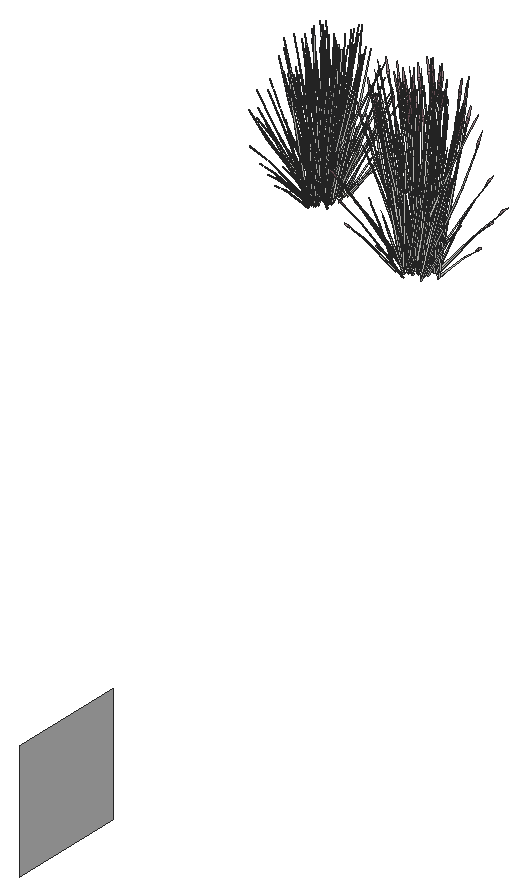
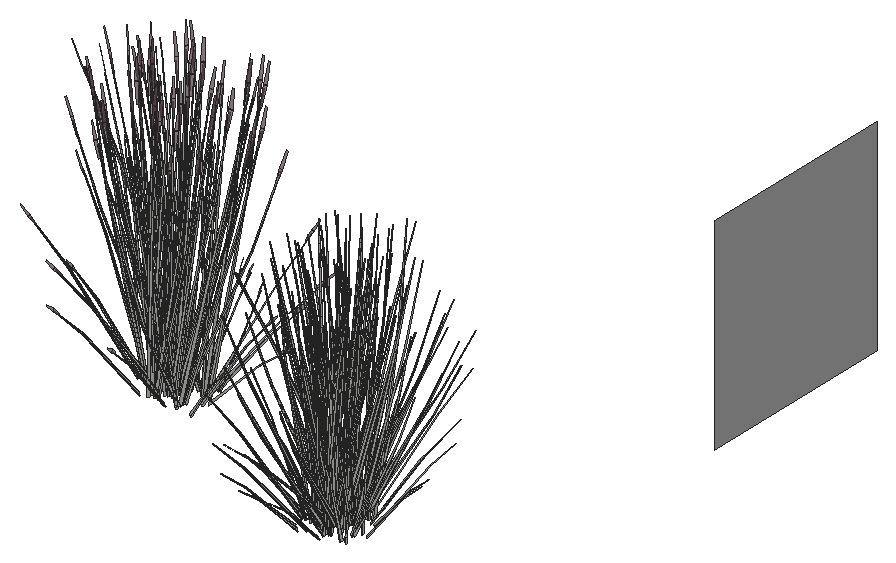
# SketchUp Ruby script. Lengths in inches.
U = 1.inch
M = Sketchup.active_model
def pt(a) = Geom::Point3d.new(a.map { |v| v * U })
def face(e, loops, mat)
  f = e.add_face(loops[0].map { |a| pt(a) })
  loops[1..].each { |l| e.add_face(l.map { |a| pt(a) }).erase! }
  f.material = f.back_material = mat if mat
  f
end
# faces: each face lists its corners as indices into pts; further lists are holes
def faces(e, pts, list, mat = nil) = list.each { |f| face(e, (f[0].is_a?(Array) ? f : [f]).map { |l| l.map { |i| pts[i] } }, mat) }
# xy, xz, yz: faces in a plane at the given z, y or x. An outline is a flat list of corners, or four numbers for a rectangle; further outlines are holes
def ring(l) = l.size == 4 ? [[l[0], l[1]], [l[2], l[1]], [l[2], l[3]], [l[0], l[3]]] : l.each_slice(2).to_a
def flat(e, list, mat, &to3) = list.each { |f| face(e, (f[0].is_a?(Array) ? f : [f]).map { |l| ring(l).map { |u, v| to3.(u, v) } }, mat) }
def xy(e, z, list, mat = nil) = flat(e, list, mat) { |x, y| [x, y, z] }
def xz(e, y, list, mat = nil) = flat(e, list, mat) { |x, z| [x, y, z] }
def yz(e, x, list, mat = nil) = flat(e, list, mat) { |y, z| [x, y, z] }
def lines(e, pts, list) = list.each { |a, b| e.add_line(pt(pts[a]), pt(pts[b])) }
# prism: a flat outline (further loops are holes) pulled along v
def prism(e, loops, v, mat = nil)
  f = face(e, loops, mat); d = Geom::Vector3d.new(v.map { |x| x * U })
  f.pushpull(f.normal.samedirection?(d) ? d.length : -d.length)
end
def box(e, o, s, mat = nil) = prism(e, [[o, [o[0] + s[0], o[1], o[2]], [o[0] + s[0], o[1] + s[1], o[2]], [o[0], o[1] + s[1], o[2]]]], [0, 0, s[2]], mat)
def at(x, y, z, deg = 0) = Geom::Transformation.translation(pt([x, y, z])) * Geom::Transformation.rotation(ORIGIN, Z_AXIS, deg.degrees)
def axes(o, x, y, z) = Geom::Transformation.new([*x, 0, *y, 0, *z, 0, *pt(o).to_a, 1])
def part(name) = M.definitions.add(name)
# library, detail: a bought-in or finely detailed component or shape, given as its bounding box
def library(name, o, s) = part(name).tap { |d| box(d.entities, o, s) }
def detail(e, o, s) = box(e.add_group.entities, o, s)
def put(e, d, t, mat = nil) = e.add_instance(d, t).tap { |i| i.material = mat if mat }
def group(e, t, mat = nil) = e.add_group.tap { |g| g.transformation = t; g.material = mat if mat }.entities
root = M.entities
M.materials.add("Glass_Mirror_01").color = [185, 185, 185]
M.materials.add("LightPink_Translucent").color = [144, 107, 117]
M.materials["LightPink_Translucent"].alpha = 0.75
c1 = part("blade")
p = [[2.15,0.21,22],[0,0.17,0],[0.09,0.45,0],[2.18,0.31,22],[2.29,0.31,22],[0.38,0.45,0],
  [2.48,0.24,33],[2.49,0.24,33],[2.48,0.22,33]]
faces(c1.entities,p,[[0,1,2,3],[4,5,2,3],[6,3,4,7],[8,0,3,6]])
c2 = part("blade with seeds\#1")
put(c2.entities,c1,at(0,0,0))
c3 = part("seeds")
p = [[0.3,-0.1,1.38],[-0.01,-0.03,1.59],[-0.01,-0.03,0.03],[0.14,-0.07,-0.07],[0.29,-0.03,3],[0.15,0.01,3.11]]
faces(c3.entities,p,[[0,1,2,3],[1,0,4,5]],"LightPink_Translucent")
c4 = part("blade with seeds")
put(c4.entities,c1,at(0,0,0))
put(c4.entities,c3,axes([2.4,0.25,30.99],[1.5799,-0.05474,1.17369],[-0.12525,1.92788,0.29478],[-0.07173,-0.02425,1.56792]))
yz(root,291,[[55.83,53.72,96.48,94.93]],"Glass_Mirror_01")
put(root,c2,axes([219.63,280.1875,145.32],[-1.0019,0.47479,-0.62955],[-0.36083,-1.36768,-0.16523],[-0.33927,0.05248,1.38963]))
put(root,c2,axes([221.34,275.85,145.32],[0.89455,-0.42392,-0.62393],[0.32217,1.22114,-0.16376],[0.30292,-0.04686,1.37722]))
put(root,c2,axes([219.46,275.97,145.28],[0.16018,-1.20264,-0.5621],[0.98808,0.25378,-0.14753],[0.11973,-0.3589,1.24074]))
put(root,c2,axes([221.5,280,145.28],[-0.16018,1.20264,-0.5621],[-0.98808,-0.25378,-0.14753],[-0.11973,0.3589,1.24074]))
put(root,c2,axes([218.61,278.11,145.28],[-0.73437,-0.77871,-0.5621],[0.66591,-0.96736,-0.14753],[-0.18319,-0.31204,1.24074]))
put(root,c2,axes([222.36,277.86,145.28],[0.73437,0.77871,-0.5621],[-0.66591,0.96736,-0.14753],[0.18319,0.31204,1.24074]))
put(root,c4,axes([263.91,261.5,146.02],[-0.50328,-1.06202,-0.69835],[1.44974,-0.38248,-0.18329],[-0.05563,-0.35963,1.54149]))
put(root,c4,axes([268.51,263.3,146.02],[0.44936,0.94823,-0.69212],[-1.29441,0.3415,-0.18165],[0.04967,0.32109,1.52773]))
put(root,c4,axes([268.38,261.3125,145.98],[1.27479,0.1698,-0.62353],[-0.26901,1.04736,-0.16365],[0.38043,0.12691,1.37633]))
put(root,c4,axes([264.11,263.48,145.98],[-1.27479,-0.1698,-0.62353],[0.26901,-1.04736,-0.16365],[-0.38043,-0.12691,1.37633]))
put(root,c4,axes([266.11,260.41,145.98],[0.82544,-0.77843,-0.62353],[1.0254,0.70586,-0.16365],[0.33076,-0.19418,1.37633]))
put(root,c4,axes([266.375,264.38,145.98],[-0.82544,0.77843,-0.62353],[-1.0254,-0.70586,-0.16365],[-0.33076,0.19418,1.37633]))
put(root,c2,axes([217.59,274.39,145.25],[0.48852,-1.08202,-0.44759],[0.87598,0.64674,0],[0.11126,-0.24644,1.41987]))
put(root,c2,axes([224.36,276.58,145.25],[0.48852,1.08202,-0.44759],[-0.87598,0.64674,0],[0.11126,0.24644,1.41987]))
put(root,c2,axes([219.49,282.99,145.25],[-0.97703,0,-0.44759],[0,-1.29348,0],[-0.22253,0,1.41987]))
put(root,c2,axes([223.375,281.58,145.25],[-0.48852,1.08202,-0.44759],[-0.87598,-0.64674,0],[-0.11126,0.24644,1.41987]))
put(root,c2,axes([216.6,279.39,145.25],[-0.48852,-1.08202,-0.44759],[0.87598,-0.64674,0],[-0.11126,-0.24644,1.41987]))
put(root,c2,axes([221.47,272.99,145.25],[0.97703,0,-0.44759],[0,1.29348,0],[0.22253,0,1.41987]))
put(root,c2,axes([219.89,279.47,145.42],[-0.88038,-0.56093,-0.40331],[0.4237,-1.16553,0.1941],[-0.20294,0,1.29492]))
put(root,c2,axes([221.1875,279.38,145.42],[-0.82007,0.69452,-0.40331],[-0.57748,-1.05199,0.1941],[-0.10147,0.22475,1.29492]))
put(root,c2,axes([219.77,276.59,145.42],[0.82007,-0.69452,-0.40331],[0.57748,1.05199,0.1941],[0.10147,-0.22475,1.29492]))
put(root,c2,axes([221.07,276.51,145.42],[0.88038,0.56093,-0.40331],[-0.4237,1.16553,0.1941],[0.20294,0,1.29492]))
put(root,c2,axes([221.78,277.9,145.42],[0.06031,1.25545,-0.40331],[-1.00118,0.11354,0.1941],[0.10147,0.22475,1.29492]))
put(root,c4,axes([270.05,259.33,145.94],[1.14694,0.51783,-0.49651],[-0.68554,0.92854,0],[0.26122,0.11794,1.57504]))
put(root,c4,axes([267.73,266.51,145.94],[-1.14694,0.51783,-0.49651],[-0.68554,-0.92854,0],[-0.26122,0.11794,1.57504]))
put(root,c4,axes([260.94,261.35,145.94],[0,-1.03566,-0.49651],[1.37109,0,0],[0,-0.23588,1.57504]))
put(root,c4,axes([262.43,265.46,145.94],[-1.14694,-0.51783,-0.49651],[0.68554,-0.92854,0],[-0.26122,-0.11794,1.57504]))
put(root,c4,axes([264.75,258.28,145.94],[1.14694,-0.51783,-0.49651],[0.68554,0.92854,0],[0.26122,-0.11794,1.57504]))
put(root,c4,axes([271.54,263.44,145.94],[0,1.03566,-0.49651],[-1.37109,0,0],[0,0.23588,1.57504]))
put(root,c2,axes([216.99,279.14,145.26],[0.24175,-1.0786,-0.27926],[0.85134,0.27158,0.27926],[-0.09817,-0.21744,1.25283]))
put(root,c2,axes([221.45,273.54,145.26],[0.60959,0.80703,-0.27926],[-0.60959,0.80703,0.27926],[0.19635,0,1.25283]))
put(root,c2,axes([223.01,281.28,145.26],[-0.85134,0.27158,-0.27926],[-0.24175,-1.0786,0.27926],[-0.09817,0.21744,1.25283]))
put(root,c2,axes([223.98,276.83,145.26],[-0.24175,1.0786,-0.27926],[-0.85134,-0.27158,0.27926],[0.09817,0.21744,1.25283]))
put(root,c2,axes([217.95,274.69,145.26],[0.85134,-0.27158,-0.27926],[0.24175,1.0786,0.27926],[0.09817,-0.21744,1.25283]))
put(root,c2,axes([219.52,282.43,145.26],[-0.60959,-0.80703,-0.27926],[0.60959,-0.80703,0.27926],[-0.19635,0,1.25283]))
put(root,c2,axes([224.54,274.45,144.77],[-0.14106,-0.08423,1.5897],[-0.41543,-1.06044,-0.24285],[0.21501,-0.3215,0.27078]))
put(root,c2,axes([220.11,283.87,144.77],[0.15398,-0.02932,1.5897],[0.80412,0.59108,-0.24285],[-0.04053,0.41985,0.27078]))
put(root,c2,axes([214.89,278.59,144.77],[0.0352,0.19392,1.5897],[-0.39624,1.07238,-0.24285],[-0.33051,-0.01799,0.27078]))
put(root,c2,axes([224.51,279.4,144.77],[-0.05317,-0.18711,1.5897],[0.29263,-1.12549,-0.24285],[0.32981,-0.03291,0.27078]))
put(root,c2,axes([220.26,271.39,144.77],[-0.14833,0.06042,1.5897],[-0.86768,-0.41907,-0.24285],[-0.01248,-0.42273,0.27078]))
put(root,c2,axes([216.1,282.05,144.77],[0.12871,0.11199,1.5897],[0.2775,1.13173,-0.24285],[-0.25244,0.2734,0.27078]))
put(root,c2,axes([224.42,284.18,144.77],[0.09761,-0.15508,1.5897],[0.90442,-0.26295,-0.24285],[0.19286,0.3437,0.27078]))
put(root,c2,axes([216.57,273.84,144.77],[-0.07697,0.17304,1.5897],[-0.85991,0.44448,-0.24285],[-0.23336,-0.29985,0.27078]))
put(root,c4,axes([264.67,261.77,146.13],[0.59459,-0.93321,-0.44739],[1.23546,0.44912,0.21531],[0,-0.21512,1.43643]))
put(root,c4,axes([264.77,263.15,146.13],[-0.73619,-0.86927,-0.44739],[1.11511,-0.61213,0.21531],[-0.23824,-0.10756,1.43643]))
put(root,c4,axes([267.72,261.65,146.13],[0.73619,0.86927,-0.44739],[-1.11511,0.61213,0.21531],[0.23824,0.10756,1.43643]))
put(root,c4,axes([267.8125,263.02,146.13],[-0.59459,0.93321,-0.44739],[-1.23546,-0.44912,0.21531],[0,0.21512,1.43643]))
put(root,c4,axes([266.34,263.77,146.13],[-1.33077,0.06393,-0.44739],[-0.12035,-1.06125,0.21531],[-0.23824,0.10756,1.43643]))
put(root,c2,axes([218.74,280.28,144.86],[0.39117,1.13797,1.16227],[-1.12236,0.3622,0.45161],[0.01867,-0.69878,1.32195]))
put(root,c2,axes([222.61,276.62,145.4],[-0.33151,-1.21377,-0.17307],[0.95493,-0.4265,0.00007],[-0.03664,-0.13398,1.56765]))
put(root,c2,axes([221.51,277.02,145.83],[1.11485,-0.13472,-0.26229],[0.06741,1.40314,-0.45076],[0.1485,0.24708,1.43974]))
put(root,c2,axes([220.34,276.37,145.83],[0.46619,-1.302,-0.26229],[0.98396,0.62692,-0.45076],[0.24158,-0.04092,1.43974]))
put(root,c2,axes([220.625,279.61,145.83],[-0.46619,1.302,-0.26229],[-0.98396,-0.62692,-0.45076],[-0.24158,0.04092,1.43974]))
put(root,c2,axes([219.46,278.95,145.83],[-1.11485,0.13472,-0.26229],[-0.06741,-1.40314,-0.45076],[-0.1485,-0.24708,1.43974]))
put(root,c2,axes([219.3125,277.33,145.83],[-0.64866,-1.16728,-0.26229],[0.91655,-0.77622,-0.45076],[0.09308,-0.288,1.43974]))
put(root,c2,axes([221.65,278.64,145.83],[0.64866,1.16728,-0.26229],[-0.91655,0.77622,-0.45076],[-0.09308,0.288,1.43974]))
put(root,c4,axes([265.02,258.69,145.95],[1.14332,0.25625,-0.30978],[-0.28787,0.90242,0.30978],[0.23049,-0.10406,1.38974]))
put(root,c4,axes([270.95,263.42,145.95],[-0.85545,0.64616,-0.30978],[-0.85545,-0.64616,0.30978],[0,0.20813,1.38974]))
put(root,c4,axes([262.75,265.07,145.95],[-0.28787,-0.90242,-0.30978],[1.14332,-0.25625,0.30978],[-0.23049,-0.10406,1.38974]))
put(root,c4,axes([267.46,266.1,145.95],[-1.14332,-0.25625,-0.30978],[0.28787,-0.90242,0.30978],[-0.23049,0.10406,1.38974]))
put(root,c4,axes([269.73,259.72,145.95],[0.28787,0.90242,-0.30978],[-1.14332,0.25625,0.30978],[0.23049,0.10406,1.38974]))
put(root,c4,axes([261.53,261.37,145.95],[0.85545,-0.64616,-0.30978],[0.85545,0.64616,0.30978],[0,-0.20813,1.38974]))
put(root,c2,axes([221.94,277.33,145.65],[-0.78639,1.12892,-0.2271],[-0.88305,-0.94994,0.49699],[0.09199,0.304,1.51643]))
put(root,c2,axes([221.66,279.28,145.625],[-1.15773,-0.30643,-0.21121],[0.20181,-1.4529,0.4622],[-0.15988,0.25387,1.41028]))
put(root,c2,axes([215.57,278.79,145.35],[0.56051,0.79893,-0.03509],[-0.61388,0.73204,-0.15911],[-0.17394,0.05154,0.52479]))
put(root,c2,axes([216.59,282.76,145.35],[0.7978,0.33351,-0.03509],[-0.24541,1.02647,-0.15911],[-0.13049,0.15585,0.52479]))
put(root,c2,axes([220.04,270.85,145.47],[-0.62476,0.71677,-0.05849],[-0.57245,-0.78502,-0.26518],[-0.0403,-0.22243,0.87466]))
put(root,c2,axes([220.87,272.21,145.21],[0.11725,0.74462,1.27635],[-0.9333,0.11852,0.07306],[-0.14126,-0.52153,0.72629]))
put(root,c4,axes([270,266.7,145.42],[0.08928,-0.14952,1.76342],[1.12407,-0.44035,-0.26939],[0.34078,0.22791,0.30037]))
put(root,c4,axes([260.01,262,145.42],[0.03108,0.16322,1.76342],[-0.62654,0.85237,-0.26939],[-0.44504,-0.04296,0.30037]))
put(root,c4,axes([265.61,256.47,145.42],[-0.20555,0.03731,1.76342],[-1.13672,-0.42002,-0.26939],[0.01907,-0.35034,0.30037]))
put(root,c4,axes([264.74,266.66,145.42],[0.19833,-0.05635,1.76342],[1.19302,0.31018,-0.26939],[0.03489,0.3496,0.30037]))
put(root,c4,axes([273.23,262.16,145.42],[-0.06405,-0.15723,1.76342],[0.44421,-0.91974,-0.26939],[0.4481,-0.01323,0.30037]))
put(root,c4,axes([261.93,257.75,145.42],[-0.11871,0.13643,1.76342],[-1.19964,0.29415,-0.26939],[-0.2898,-0.26759,0.30037]))
put(root,c4,axes([259.67,266.57,145.42],[0.16438,0.10347,1.76342],[0.27873,0.95868,-0.26939],[-0.36432,0.20444,0.30037]))
put(root,c4,axes([270.64,258.25,145.42],[-0.18342,-0.08159,1.76342],[-0.47115,-0.9115,-0.26939],[0.31784,-0.24736,0.30037]))
put(root,c2,axes([216.75,280.375,145.57],[-0.97904,0.72283,0],[-0.54599,-1.20931,-0.46523],[-0.12435,-0.27543,1.47583]))
put(root,c2,axes([223.96,280.92,145.57],[0.97904,0.72283,0],[-0.54599,1.20931,-0.46523],[-0.12435,0.27543,1.47583]))
put(root,c2,axes([224.21,275.6,145.57],[0.97904,-0.72283,0],[0.54599,1.20931,-0.46523],[0.12435,0.27543,1.47583]))
put(root,c2,axes([220.23,283.31,145.57],[0,1.44565,0],[-1.09198,0,-0.46523],[-0.24871,0,1.47583]))
put(root,c2,axes([222.76,277.39,145.49],[1.12244,-0.50265,-0.0542],[0.39331,1.43622,0],[0.0392,-0.01755,1.55211]))
put(root,c2,axes([217,275.05,145.57],[-0.97904,-0.72283,0],[0.54599,-1.20931,-0.46523],[0.12435,-0.27543,1.47583]))
put(root,c2,axes([220.73,272.66,145.57],[0,-1.44565,0],[1.09198,0,-0.46523],[0.24871,0,1.47583]))
put(root,c2,axes([221,277.0625,145.5],[-0.84094,1.07538,-0.05527],[-0.84146,-1.07603,0],[-0.02937,0.03755,1.58274]))
put(root,c2,axes([220.57,276.7,145.49],[1.12994,0,-0.05082],[0,1.44565,0],[0.03551,0,1.61697]))
put(root,c2,axes([224.1,276.51,145.4],[-0.98246,0.71382,-0.04636],[-0.54599,-1.20931,0.46523],[0.09354,0.298,1.4751]))
put(root,c2,axes([221.29,273.24,145.41],[-0.00781,1.44494,-0.04486],[-1.09198,0,0.45022],[0.24858,0.04541,1.42752]))
put(root,c2,axes([219.95,282.1875,145.53],[0.82143,1.07538,0.27726],[-0.81279,1.07603,-0.32897],[-0.23327,0.03755,1.48641]))
put(root,c2,axes([223.6,276.48,145.53],[0.31757,-1.44738,0.27726],[1.13512,0.3621,-0.32897],[0.14207,0.23956,1.48641]))
put(root,c2,axes([223.11,278.29,145.41],[-0.43865,1.16553,0],[-0.91144,-0.56093,0],[0,0,1.46678]))
put(root,c2,axes([222.73,278.03,145.41],[-0.84234,0.37722,0],[-0.29498,-1.07717,0],[0,0,1.39163]))
put(root,c2,axes([223.13,276.97,145.41],[0.43865,-1.16553,0],[0.91144,0.56093,0],[0,0,1.57718]))
put(root,c2,axes([220.125,277.43,145.42],[-1.1305,0,0],[0,-1.44565,0],[0,0,1.61777]))
put(root,c2,axes([220.375,276.45,145.42],[0,-1.29348,0],[1.0115,0,0],[0,0,1.60831]))
put(root,c2,axes([220.81,276.47,145.42],[0.63109,-0.80703,0],[0.63109,0.80703,0],[0,0,1.52591]))
put(root,c4,axes([263.81,260.54,145.52],[-1.20625,0.41464,1.28929],[-0.38394,-1.1897,0.50096],[0.74071,0.01979,1.46642]))
put(root,c4,axes([267.27,263.48,146.59],[0.1428,1.18174,-0.29095],[-1.48733,0.07145,-0.50002],[-0.26191,0.15741,1.59708]))
put(root,c4,axes([267.96,262.24,146.59],[1.38012,0.49416,-0.29095],[-0.66454,1.04299,-0.50002],[0.04337,0.25608,1.59708]))
put(root,c4,axes([264.53,262.55,146.59],[-1.38012,-0.49416,-0.29095],[0.66454,-1.04299,-0.50002],[-0.04337,-0.25608,1.59708]))
put(root,c4,axes([265.22,261.31,146.59],[-0.1428,-1.18174,-0.29095],[1.48733,-0.07145,-0.50002],[0.26191,-0.15741,1.59708]))
put(root,c4,axes([266.93,261.16,146.59],[1.23732,-0.68758,-0.29095],[0.8228,0.97154,-0.50002],[0.30528,0.09867,1.59708]))
put(root,c4,axes([265.55,263.63,146.59],[-1.23732,0.68758,-0.29095],[-0.8228,-0.97154,-0.50002],[-0.30528,-0.09867,1.59708]))
put(root,c4,axes([267.69,264.66,146.11],[1.2866,-0.3514,-0.19198],[0.45209,1.01223,0.00008],[0.14202,-0.03884,1.73897]))
put(root,c2,axes([221.1,279.11,145.56],[0.20585,-1.46124,0.41247],[1.16261,0.29738,0.16186],[-0.11226,0.21355,1.43206]))
put(root,c2,axes([219.41,278.11,145.56],[0.88667,0.95859,0.41247],[-0.7827,1.13884,0.16186],[-0.08849,-0.2311,1.43206]))
put(root,c2,axes([220.03,279.23,145.56],[1.09253,-0.50265,0.41247],[0.37991,1.43622,0.16186],[-0.20075,-0.01755,1.43206]))
put(root,c2,axes([219.86,276.86,145.57],[-0.20585,1.46124,0.44352],[-1.16261,-0.29738,0.17404],[0.11226,-0.21355,1.53985]))
put(root,c2,axes([221.72,276.76,145.79],[0.58702,-0.85413,0.13053],[0.66228,0.71246,-0.37274],[0.08953,0.19831,1.14258]))
put(root,c2,axes([219.03,277.22,145.79],[-0.87196,-0.22303,0.13053],[0.15136,-1.08968,-0.37274],[0.08953,-0.19831,1.14258]))
put(root,c2,axes([220.27,276,145.79],[-0.28493,-1.07717,0.13053],[0.81364,-0.37722,-0.37274],[0.17907,0,1.14258]))
put(root,c2,axes([221.93,278.75,145.79],[0.87196,0.22303,0.13053],[-0.15136,1.08968,-0.37274],[-0.08953,0.19831,1.14258]))
put(root,c2,axes([224.64,281.99,145.97],[-0.17302,-1.05027,0.05866],[0.69705,-0.24145,-0.77802],[0.35285,0.06658,0.69739]))
put(root,c2,axes([218.28,283.0625,145.76],[0.27202,-0.22572,1.28914],[0.7394,0.52014,-0.27724],[-0.17673,0.53408,0.55117]))
put(root,c2,axes([225.38,282.24,145.76],[-0.15413,-0.36483,1.28914],[0.46474,-0.90077,-0.27724],[0.40213,0.2681,0.55117]))
put(root,c2,axes([223.2,276.95,145.76],[-0.32388,-0.0204,1.28914],[-0.36177,-0.97496,-0.27724],[0.38765,-0.30097,0.55117]))
put(root,c2,axes([215.96,276.14,145.76],[0.19776,0.32863,1.28914],[-0.34614,0.98419,-0.27724],[-0.43048,-0.18244,0.55117]))
put(root,c2,axes([218.29,272.97,145.76],[-0.02894,0.41302,1.28914],[-0.77632,0.42312,-0.27724],[-0.21961,-0.50739,0.55117]))
put(root,c2,axes([215.59,281.22,145.76],[0.31962,0.07001,1.28914],[0.26756,1.02347,-0.27724],[-0.41311,0.23924,0.55117]))
put(root,c2,axes([222.25,272,145.76],[-0.2403,0.27843,1.28914],[-0.79492,-0.36227,-0.27724],[0.10768,-0.56334,0.55117]))
put(root,c2,axes([222.25,284.62,145.76],[0.08021,-0.40179,1.28914],[0.81924,-0.25896,-0.27724],[0.15335,0.54576,0.55117]))
put(root,c4,axes([266.94,263.95,146.39],[-1.19666,-0.83357,-0.25192],[1.00694,-0.93603,0.5513],[-0.32224,0.09751,1.68216]))
put(root,c2,axes([220.4,282.43,145.66],[0.97703,0,0.44759],[0,1.29348,0],[-0.22253,0,1.41987]))
put(root,c2,axes([217.51,275.67,145.66],[-0.48852,1.08202,0.44759],[-0.87598,-0.64674,0],[0.11126,-0.24644,1.41987]))
put(root,c2,axes([220.5625,273.54,145.66],[-0.97703,0,0.44759],[0,-1.29348,0],[0.22253,0,1.41987]))
put(root,c2,axes([223.53,275.85,145.66],[-0.48852,-1.08202,0.44759],[0.87598,-0.64674,0],[0.11126,0.24644,1.41987]))
put(root,c2,axes([223.45,280.3,145.66],[0.48852,-1.08202,0.44759],[0.87598,0.64674,0],[-0.11126,0.24644,1.41987]))
put(root,c4,axes([264.875,263.64,146.36],[0.32481,-1.2272,-0.23429],[1.54007,0.21392,0.51271],[-0.26911,-0.16947,1.5644]))
put(root,c2,axes([220.33,278.77,145.62],[0.47355,-1.30265,0.21694],[0.98396,0.62692,0.45076],[-0.22682,0,1.44726]))
put(root,c2,axes([218,276.08,145.66],[0.25932,1.24233,0.15904],[-0.96507,0.30677,0.3163],[0.14061,-0.1108,1.44604]))
put(root,c2,axes([220.53,274.29,145.66],[-0.71168,0.90835,0.15904],[-0.69029,-0.91538,0.3163],[0.14534,0.10032,1.44604]))
put(root,c2,axes([217.95,279.78,145.66],[0.971,0.33398,0.15904],[-0.27478,1.22215,0.3163],[-0.00473,-0.21112,1.44604]))
put(root,c2,axes([223.01,276.2,145.66],[-0.971,-0.33398,0.15904],[0.27478,-1.22215,0.3163],[0.00473,0.21112,1.44604]))
put(root,c2,axes([222.96,279.89,145.66],[-0.25932,-1.24233,0.15904],[0.96507,-0.30677,0.3163],[-0.14061,0.1108,1.44604]))
put(root,c2,axes([220.07,276.48,145.88],[-0.88038,-0.56093,0.40331],[0.4237,-1.16553,-0.1941],[0.20294,0,1.29492]))
put(root,c2,axes([219.67,279.19,145.88],[0.06031,1.25545,0.40331],[-1.00118,0.11354,-0.1941],[-0.10147,-0.22475,1.29492]))
put(root,c2,axes([219.26,277.69,145.88],[-0.82007,0.69452,0.40331],[-0.57748,-1.05199,-0.1941],[0.10147,-0.22475,1.29492]))
put(root,c2,axes([220.89,279.49,145.88],[0.88038,0.56093,0.40331],[-0.4237,1.16553,-0.1941],[-0.20294,0,1.29492]))
put(root,c2,axes([221.29,276.78,145.88],[-0.06031,-1.25545,0.40331],[1.00118,-0.11354,-0.1941],[0.10147,0.22475,1.29492]))
put(root,c4,axes([265.39,257.19,146.05],[-0.84686,0.59414,-0.03893],[-0.77596,-0.65071,-0.17649],[-0.05463,-0.18438,0.58215]))
put(root,c4,axes([261.18,258.27,146.05],[-0.35352,0.84566,-0.03893],[-1.08806,-0.26014,-0.17649],[-0.1652,-0.13832,0.58215]))
put(root,c4,axes([273.81,261.93,146.19],[-0.75977,-0.66224,-0.06488],[0.83212,-0.6068,-0.29416],[0.23578,-0.04272,0.97024]))
put(root,c4,axes([272.37,262.81,145.91],[-0.7893,0.12429,1.41583],[-0.12563,-0.9893,0.08104],[0.55282,-0.14974,0.80566]))
put(root,c2,axes([224.77,274.52,145.83],[-0.03064,0.74138,0.9471],[-0.6508,-0.48961,0.52291],[0.23122,-0.29288,0.74292]))
put(root,c4,axes([267.81,266.23,146.12],[-0.75665,-1.04141,-0.05142],[1.28187,-0.57875,0.51607],[-0.31588,0.09915,1.6363]))
put(root,c4,axes([271.27,263.25,146.125],[-1.53164,-0.00828,-0.04976],[0,-1.1575,0.49943],[-0.04813,0.2635,1.58352]))
put(root,c4,axes([266.875,264.8125,146.22],[0.53281,1.18979,-0.06012],[-1.52239,0.41691,0],[0.01861,0.04155,1.72173]))
put(root,c4,axes([267.22,262.94,146.22],[-1.1399,-0.8914,-0.06131],[1.1406,-0.89194,0],[-0.03981,-0.03113,1.75571]))
put(root,c2,axes([219.1,284.41,145.92],[-0.06991,-0.73811,1.03545],[0.616,0.4682,0.76078],[-0.09241,0.36475,0.22807]))
put(root,c2,axes([223.5,274.63,145.92],[-0.28093,0.65095,1.03545],[-0.28545,-0.84053,0.76078],[0.2418,-0.22671,0.22807]))
put(root,c2,axes([223.96,285.45,145.92],[-0.44281,-0.48182,1.03545],[0.70101,-0.19012,0.76078],[0.12552,0.34819,0.22807]))
put(root,c2,axes([221.1875,270.66,145.92],[0.1613,0.71432,1.03545],[-0.66662,-0.33623,0.76078],[0.04561,-0.37895,0.22807]))
put(root,c2,axes([215.07,281.58,145.92],[0.34005,-0.60308,1.03545],[0.20441,0.87829,0.76078],[-0.26134,0.18792,0.22807]))
put(root,c2,axes([225.9,281.37,145.92],[-0.58095,0.02992,1.03545],[0.41436,-0.74764,0.76078],[0.2769,0.14704,0.22807]))
put(root,c2,axes([216.86,272.49,145.92],[0.49736,0.38508,1.03545],[-0.66822,0.331,0.76078],[-0.16744,-0.31805,0.22807]))
put(root,c2,axes([214.39,277.35,145.92],[0.56973,-0.14831,1.03545],[-0.31555,0.82274,0.76078],[-0.29172,-0.08853,0.22807]))
put(root,c4,axes([267.61,262.49,146.22],[0,1.19774,-0.05637],[-1.53239,0,0],[0,0.03764,1.79368]))
put(root,c4,axes([263.71,258.44,146.3],[-0.7662,-1.03778,0],[1.28187,-0.57875,-0.51607],[0.29196,-0.13181,1.63711]))
put(root,c4,axes([263.13,266.09,146.3],[-0.7662,1.03778,0],[-1.28187,-0.57875,-0.51607],[-0.29196,-0.13181,1.63711]))
put(root,c4,axes([268.77,266.35,146.3],[0.7662,1.03778,0],[-1.28187,0.57875,-0.51607],[-0.29196,0.13181,1.63711]))
put(root,c4,axes([260.6,262.13,146.3],[-1.53239,0,0],[0,-1.1575,-0.51607],[0,-0.26363,1.63711]))
put(root,c4,axes([269.35,258.71,146.3],[0.7662,-1.03778,0],[1.28187,0.57875,-0.51607],[0.29196,0.13181,1.63711]))
put(root,c4,axes([271.89,262.66,146.3],[1.53239,0,0],[0,1.1575,-0.51607],[0,0.26363,1.63711]))
put(root,c2,axes([220.33,276.21,145.99],[-0.91991,0.03158,1.27354],[0.23846,-1.42935,0.53923],[0.50337,0.33806,1.20213]))
put(root,c4,axes([261.79,261.83,146.25],[-1.1399,0.87071,0.30756],[-1.1406,-0.86155,-0.36492],[-0.03981,-0.24727,1.64885]))
put(root,c4,axes([267.84,265.7,146.25],[1.53422,0.33662,0.30756],[-0.38383,1.20322,-0.36492],[-0.25393,0.15059,1.64885]))
put(root,c4,axes([265.92,265.18,146.12],[-1.23546,-0.46496,0],[0.59459,-0.96613,0],[0,0,1.62707]))
put(root,c4,axes([267.32,265.2,146.13],[1.23546,0.46496,0],[-0.59459,0.96613,0],[0,0,1.74954]))
put(root,c4,axes([266.2,264.78,146.13],[-0.39985,-0.89288,0],[1.1418,-0.31268,0],[0,0,1.54371]))
put(root,c4,axes([266.84,262.02,146.13],[0,-1.19833,0],[1.53239,0,0],[0,0,1.79456]))
put(root,c4,axes([267.875,262.28,146.13],[1.37109,0,0],[0,1.07219,0],[0,0,1.78407]))
put(root,c4,axes([267.85,262.74,146.14],[0.85545,0.66896,0],[-0.85545,0.66896,0],[0,0,1.69266]))
put(root,c4,axes([265.05,263.05,146.29],[1.54892,0.2182,0.45755],[-0.31522,1.23236,0.17955],[-0.22636,-0.119,1.58856]))
put(root,c4,axes([266.11,261.26,146.29],[-1.01611,0.93987,0.45755],[-1.20717,-0.82966,0.17955],[0.24496,-0.0938,1.58856]))
put(root,c4,axes([264.92,261.92,146.29],[0.53281,1.15808,0.45755],[-1.52239,0.4027,0.17955],[0.01861,-0.2128,1.58856]))
put(root,c4,axes([267.43,261.74,146.31],[-1.54892,-0.2182,0.49198],[0.31522,-1.23236,0.19306],[0.22636,0.119,1.70813]))
put(root,c2,axes([216.875,280.12,147.92],[-0.47225,0.98582,-0.64046],[-0.82754,-0.7006,0.07729],[-0.28197,0.35717,0.906]))
put(root,c2,axes([224.13,279.05,147.92],[0.79444,-0.5518,-0.64046],[0.44274,1.13586,0.07729],[0.38385,-0.12903,0.906]))
put(root,c2,axes([218.04,282.13,147.92],[-0.02352,1.1557,-0.64046],[-0.99061,-0.07762,0.07729],[-0.10454,0.48961,0.906]))
put(root,c2,axes([219,273.85,147.92],[-0.77091,-0.6039,-0.64046],[0.54787,-1.05824,0.07729],[-0.27931,-0.36058,0.906]))
put(root,c2,axes([220.94,273.56,147.92],[-0.4315,-1.0159,-0.64046],[0.88824,-0.56616,0.07729],[-0.1009,-0.49086,0.906]))
put(root,c2,axes([217.43,275.34,147.92],[-0.90375,-0.03008,-0.64046],[0.0607,-1.26677,0.07729],[-0.38287,-0.13368,0.906]))
put(root,c2,axes([222.74,274.55,147.92],[0.02352,-1.1557,-0.64046],[0.99061,0.07762,0.07729],[0.10454,-0.48961,0.906]))
put(root,c2,axes([216.65,277.64,147.92],[-0.79444,0.5518,-0.64046],[-0.44274,-1.13586,0.07729],[-0.38385,0.12903,0.906]))
put(root,c2,axes([224.29,278.63,147.65],[0.24493,-1.13649,-0.46065],[0.83975,0.38955,-0.35681],[0.33809,-0.10421,0.88141]))
put(root,c2,axes([217.125,275.59,147.65],[-0.65648,0.82762,-0.46065],[-0.57493,-0.87428,-0.35681],[-0.33354,-0.12593,0.88141]))
put(root,c2,axes([216.9,280.58,147.65],[0.23225,1.14083,-0.46065],[-0.87956,0.19957,-0.35681],[-0.25205,0.30642,0.88141]))
put(root,c2,axes([220.62,273.35,147.65],[-0.88873,-0.31321,-0.46065],[0.30463,-1.07385,-0.35681],[-0.08149,-0.43235,0.88141]))
put(root,c2,axes([218.24,282.51,147.65],[0.6472,0.83949,-0.46065],[-0.68369,0.73521,-0.35681],[-0.09847,0.42653,0.88141]))
put(root,c2,axes([222.14,282.81,147.65],[0.89213,-0.297,-0.46065],[0.15606,1.12475,-0.35681],[0.23962,0.32232,0.88141]))
put(root,c2,axes([220.16,283.33,147.65],[0.88873,0.31321,-0.46065],[-0.30463,1.07385,-0.35681],[0.08149,0.43235,0.88141]))
put(root,c2,axes([216.49,278.05,147.65],[-0.24493,1.13649,-0.46065],[-0.83975,-0.38955,-0.35681],[-0.33809,0.10421,0.88141]))
put(root,c2,axes([218.64,273.875,147.65],[-0.89213,0.297,-0.46065],[-0.15606,-1.12475,-0.35681],[-0.23962,-0.32232,0.88141]))
put(root,c2,axes([223.88,276.1,147.65],[-0.23225,-1.14083,-0.46065],[0.87956,-0.19957,-0.35681],[0.25205,-0.30642,0.88141]))
put(root,c4,axes([265.41,262.23,146.36],[1.3808,0.50196,0.24065],[-0.66454,1.04299,0.50002],[0,-0.24043,1.60543]))
put(root,c4,axes([267.54,263.71,146.54],[0.90538,0.62224,0.1448],[-0.75521,0.70202,-0.41347],[-0.21021,0.09491,1.26744]))
put(root,c4,axes([267.05,260.86,146.54],[0.23642,-0.92427,0.1448],[1.15506,0.16044,-0.41347],[0.21021,0.09491,1.26744]))
put(root,c4,axes([268.35,262.17,146.54],[1.1418,-0.30203,0.1448],[0.39985,0.86246,-0.41347],[0,0.18981,1.26744]))
put(root,c4,axes([265.43,263.93,146.54],[-0.23642,0.92427,0.1448],[-1.15506,-0.16044,-0.41347],[-0.21021,-0.09491,1.26744]))
put(root,c4,axes([262,266.8,146.75],[1.11329,-0.1834,0.06507],[0.25594,0.73887,-0.86304],[-0.07058,0.37403,0.7736]))
put(root,c4,axes([260.86,260.07,146.52],[0.23927,0.28834,1.43002],[-0.55135,0.78376,-0.30754],[-0.56612,-0.18733,0.61141]))
put(root,c4,axes([261.73,267.59,146.52],[0.38672,-0.16338,1.43002],[0.95481,0.49262,-0.30754],[-0.28419,0.42626,0.61141]))
put(root,c4,axes([267.35,265.27,146.52],[0.02163,-0.34331,1.43002],[1.03345,-0.38348,-0.30754],[0.31903,0.4109,0.61141]))
put(root,c4,axes([268.2,257.6,146.52],[-0.34835,0.20963,1.43002],[-1.04325,-0.36691,-0.30754],[0.19338,-0.4563,0.61141]))
put(root,c4,axes([271.56,260.07,146.52],[-0.4378,-0.03068,1.43002],[-0.44851,-0.8229,-0.30754],[0.53783,-0.23279,0.61141]))
put(root,c4,axes([262.81,257.21,146.52],[-0.07421,0.33879,1.43002],[-1.08488,0.28361,-0.30754],[-0.25359,-0.4379,0.61141]))
put(root,c4,axes([272.59,264.28,146.52],[-0.29514,-0.25472,1.43002],[0.38401,-0.84262,-0.30754],[0.59714,0.11414,0.61141]))
put(root,c4,axes([259.22,264.27,146.52],[0.42589,0.08502,1.43002],[0.2745,0.86839,-0.30754],[-0.57851,0.16255,0.61141]))
put(root,c4,axes([268.26,259.77,146.4],[-1.31687,0.27488,0.17642],[-0.32517,-1.02297,0.35086],[0.11745,0.14905,1.60407]))
put(root,c4,axes([270.16,262.45,146.4],[-0.96285,-0.75439,0.17642],[0.97031,-0.7317,0.35086],[-0.10634,0.15406,1.60407]))
put(root,c4,axes([264.35,259.71,146.4],[-0.35402,1.02926,0.17642],[-1.29548,-0.29127,0.35086],[0.22379,-0.00501,1.60407]))
put(root,c4,axes([268.14,265.08,146.4],[0.35402,-1.02926,0.17642],[1.29548,0.29127,0.35086],[-0.22379,0.00501,1.60407]))
put(root,c4,axes([264.22,265.02,146.4],[1.31687,-0.27488,0.17642],[0.32517,1.02297,0.35086],[-0.11745,-0.14905,1.60407]))
put(root,c4,axes([261.53,262.31,146.4],[0,1.03566,0.49651],[-1.37109,0,0],[0,-0.23588,1.57504]))
put(root,c4,axes([268.69,259.25,146.4],[-1.14694,-0.51783,0.49651],[0.68554,-0.92854,0],[0.26122,0.11794,1.57504]))
put(root,c4,axes([270.96,262.48,146.4],[0,-1.03566,0.49651],[1.37109,0,0],[0,0.23588,1.57504]))
put(root,c4,axes([268.5,265.63,146.4],[1.14694,-0.51783,0.49651],[0.68554,0.92854,0],[-0.26122,0.11794,1.57504]))
put(root,c4,axes([263.79,265.54,146.4],[1.14694,0.51783,0.49651],[-0.68554,0.92854,0],[-0.26122,-0.11794,1.57504]))
put(root,c2,axes([219.625,281.0625,146.44],[-0.14134,-0.32863,1.5962],[0.98684,-0.11332,0.12492],[0.13095,0.71181,0.57049]))
put(root,c2,axes([223.35,281.34,148.24],[0.90375,0.03008,-0.71091],[-0.0607,1.26677,0.08579],[0.38287,0.13368,1.00565]))
